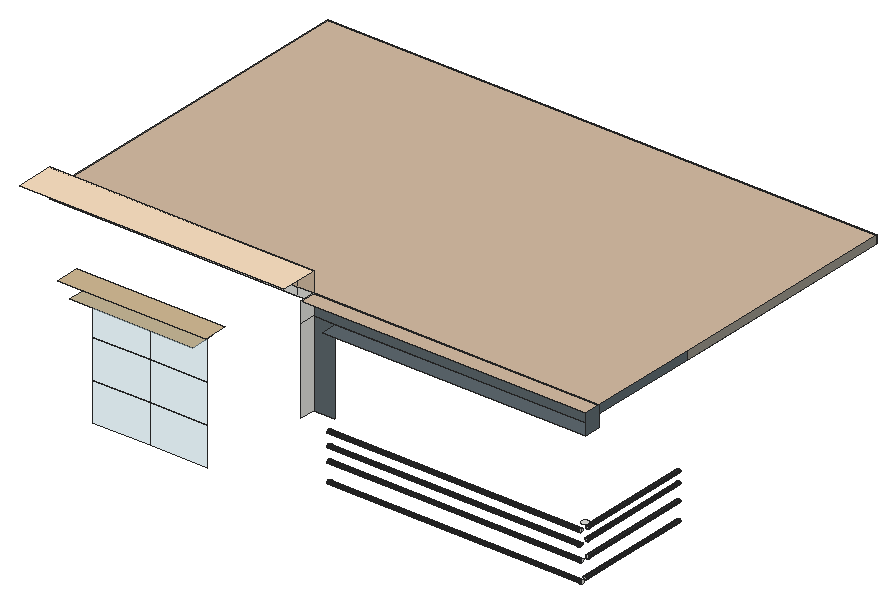
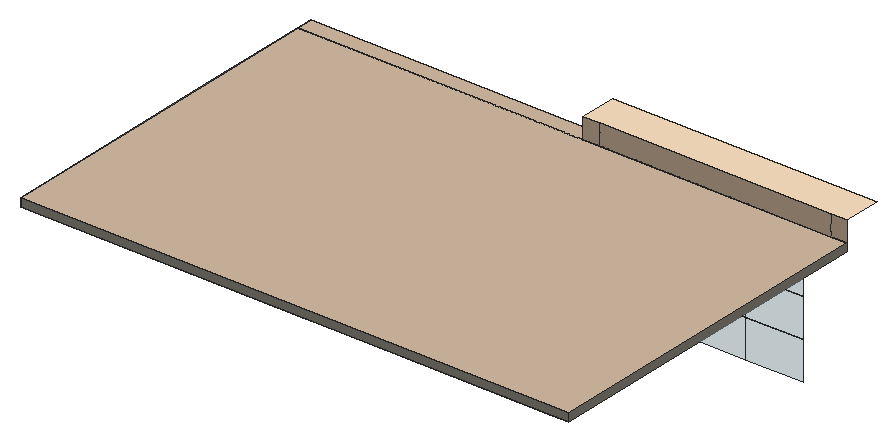
# SketchUp Ruby script. Lengths in inches.
U = 1.inch
M = Sketchup.active_model
def pt(a) = Geom::Point3d.new(a.map { |v| v * U })
def face(e, loops, mat)
  f = e.add_face(loops[0].map { |a| pt(a) })
  loops[1..].each { |l| e.add_face(l.map { |a| pt(a) }).erase! }
  f.material = f.back_material = mat if mat
  f
end
# faces: each face lists its corners as indices into pts; further lists are holes
def faces(e, pts, list, mat = nil) = list.each { |f| face(e, (f[0].is_a?(Array) ? f : [f]).map { |l| l.map { |i| pts[i] } }, mat) }
# xy, xz, yz: faces in a plane at the given z, y or x. An outline is a flat list of corners, or four numbers for a rectangle; further outlines are holes
def ring(l) = l.size == 4 ? [[l[0], l[1]], [l[2], l[1]], [l[2], l[3]], [l[0], l[3]]] : l.each_slice(2).to_a
def flat(e, list, mat, &to3) = list.each { |f| face(e, (f[0].is_a?(Array) ? f : [f]).map { |l| ring(l).map { |u, v| to3.(u, v) } }, mat) }
def xy(e, z, list, mat = nil) = flat(e, list, mat) { |x, y| [x, y, z] }
def xz(e, y, list, mat = nil) = flat(e, list, mat) { |x, z| [x, y, z] }
def yz(e, x, list, mat = nil) = flat(e, list, mat) { |y, z| [x, y, z] }
def lines(e, pts, list) = list.each { |a, b| e.add_line(pt(pts[a]), pt(pts[b])) }
# prism: a flat outline (further loops are holes) pulled along v
def prism(e, loops, v, mat = nil)
  f = face(e, loops, mat); d = Geom::Vector3d.new(v.map { |x| x * U })
  f.pushpull(f.normal.samedirection?(d) ? d.length : -d.length)
end
def box(e, o, s, mat = nil) = prism(e, [[o, [o[0] + s[0], o[1], o[2]], [o[0] + s[0], o[1] + s[1], o[2]], [o[0], o[1] + s[1], o[2]]]], [0, 0, s[2]], mat)
def at(x, y, z, deg = 0) = Geom::Transformation.translation(pt([x, y, z])) * Geom::Transformation.rotation(ORIGIN, Z_AXIS, deg.degrees)
def axes(o, x, y, z) = Geom::Transformation.new([*x, 0, *y, 0, *z, 0, *pt(o).to_a, 1])
def part(name) = M.definitions.add(name)
# library, detail: a bought-in or finely detailed component or shape, given as its bounding box
def library(name, o, s) = part(name).tap { |d| box(d.entities, o, s) }
def detail(e, o, s) = box(e.add_group.entities, o, s)
def put(e, d, t, mat = nil) = e.add_instance(d, t).tap { |i| i.material = mat if mat }
def group(e, t, mat = nil) = e.add_group.tap { |g| g.transformation = t; g.material = mat if mat }.entities
root = M.entities
M.materials.add("[0012_Bisque]").color = [255, 228, 196]
M.materials.add("[Color M07]").color = [58, 58, 58]
M.materials.add("[Formica Beige]").color = [211, 187, 149]
M.materials.add("[Formica Graystone]").color = [149, 146, 135]
M.materials.add("[Formica Laminate Light]").color = [213, 189, 164]
M.materials.add("[Formica Speckled Grey]").color = [94, 105, 111]
M.materials.add("[Quartz Light Brown]").color = [199, 184, 152]
M.materials.add("[Translucent Glass Safety]").color = [204, 235, 244]
M.materials["[Translucent Glass Safety]"].alpha = 0.5
c1 = library("Group\#1",[-0.5,-0.5,-0.1],[10.11,10.11,0.2])
c2 = library("Group\#2",[-0.5,-0.5,-0.1],[10.11,10.11,0.2])
c3 = library("Group\#3",[-0.5,-0.5,-0.1],[10.11,10.11,0.2])
c4 = library("Group\#4",[-0.5,-0.5,-0.1],[10.11,10.11,0.2])
xy(root,170.34,[[254.97,24.03,255.38,24.08,255.75,24.24,256.08,24.49,256.33,24.8125,256.48,25.19,256.54,25.59,256.48,26,256.33,26.375,256.08,26.7,255.75,26.95,255.38,27.1,254.97,27.16,254.57,27.1,254.19,26.95,253.87,26.7,253.62,26.375,253.46,26,253.41,25.59,253.46,25.19,253.62,24.8125,253.87,24.49,254.19,24.24,254.57,24.08]])
xy(root,197.75,[[32.29,0,90.53,11.1875]],"[Quartz Light Brown]")
xy(root,203.54,[[26.5,0,96.3125,11.1875]],"[Formica Beige]")
xy(root,210.1875,[[134.6,21.1875,259.04,28.73]],"[Formica Speckled Grey]")
xy(root,216.125,[[0,28.73,7.54,80.93],[7.54,28.73,116.61,80.93],[116.61,28.73,124.35,80.93],[0,80.93,7.54,89.9],[7.54,80.93,116.61,89.9],
  [116.61,80.93,124.35,89.9],[124.35,80.93,251.5,89.9],[251.5,80.93,259.04,89.9],[0,89.9,7.54,192.39],[7.54,89.9,116.61,184.85],
  [116.61,89.9,124.35,184.85],[124.35,89.9,251.5,184.85],[251.5,89.9,259.04,184.85],[7.54,184.85,116.61,192.39],[116.61,184.85,124.35,192.39],
  [124.35,184.85,259.04,192.39]])
xy(root,216.125,[[124.35,28.73,259.04,80.93]],"[Formica Speckled Grey]")
xy(root,219.875,[[124.35,21.1875,259.04,28.73],[0,28.73,259.04,192.39]],"[Formica Laminate Light]")
xy(root,229.5,[[0,11.1875,124.35,28.73]],"[0012_Bisque]")
xz(root,11.1875,[[34.45,140.9,61.41,159.07],[61.41,140.9,88.37,159.07],[34.45,159.07,61.41,177.24],[61.41,159.07,88.37,177.24],[34.45,177.24,61.41,195.59],
  [61.41,177.24,88.37,195.59]],"[Translucent Glass Safety]")
xz(root,25.59,[[254.99,145.96,255.2,145.99,255.39,146.07,255.5625,146.2,255.69,146.37,255.77,146.5625,255.8,146.77,255.77,146.98,255.69,147.18,255.5625,147.35,255.39,147.48,255.2,147.56,254.99,147.58,254.78,147.56,254.58,147.48,254.41,147.35,254.28,147.18,254.2,146.98,254.18,146.77,254.2,146.5625,254.28,146.37,254.41,146.2,254.58,146.07,254.78,145.99]])
xz(root,26.7,[[254.99,161.79,255.2,161.81,255.39,161.9,255.5625,162.03,255.69,162.19,255.77,162.39,255.8,162.6,255.77,162.81,255.69,163.01,255.5625,163.17,255.39,163.3,255.2,163.38,254.99,163.41,254.78,163.38,254.58,163.3,254.41,163.17,254.28,163.01,254.2,162.81,254.18,162.6,254.2,162.39,254.28,162.19,254.41,162.03,254.58,161.9,254.78,161.81]])
xz(root,26.99,[[254.99,166.97,255.2,167,255.39,167.08,255.5625,167.21,255.69,167.38,255.77,167.58,255.8,167.79,255.77,168,255.69,168.19,255.5625,168.36,255.39,168.49,255.2,168.57,254.99,168.6,254.78,168.57,254.58,168.49,254.41,168.36,254.28,168.19,254.2,168,254.18,167.79,254.2,167.58,254.28,167.38,254.41,167.21,254.58,167.08,254.78,167]])
xz(root,27.05,[[254.99,154.29,255.2,154.31,255.39,154.4,255.5625,154.53,255.69,154.69,255.77,154.89,255.8,155.1,255.77,155.31,255.69,155.51,255.5625,155.67,255.39,155.8,255.2,155.88,254.99,155.91,254.78,155.88,254.58,155.8,254.41,155.67,254.28,155.51,254.2,155.31,254.18,155.1,254.2,154.89,254.28,154.69,254.41,154.53,254.58,154.4,254.78,154.31]])
xz(root,28.73,[[0,216.125,116.61,219.875],[116.61,216.125,124.35,219.875],[124.35,216.125,259.04,219.875]])
xz(root,28.73,[[0,219.875,7.54,229.5],[7.54,219.875,116.61,229.5],[116.61,219.875,124.35,229.5]],"[Formica Laminate Light]")
xz(root,28.73,[[124.35,170.34,134.6,210.1875],[124.35,210.1875,259.04,216.125]],"[Formica Speckled Grey]")
xz(root,192.39,[[0,216.125,259.04,219.875]],"[Formica Graystone]")
yz(root,0,[[28.73,216.125,192.39,219.875]],"[Formica Graystone]")
yz(root,124.35,[[21.1875,170.34,28.73,210.1875],[21.1875,210.1875,28.73,219.875]])
yz(root,253.78,[[24.83,159.95,25.04,159.97,25.23,160.05,25.4,160.18,25.53,160.35,25.61,160.55,25.64,160.76,25.61,160.97,25.53,161.16,25.4,161.33,25.23,161.46,25.04,161.54,24.83,161.57,24.62,161.54,24.42,161.46,24.25,161.33,24.125,161.16,24.04,160.97,24.01,160.76,24.04,160.55,24.125,160.35,24.25,160.18,24.42,160.05,24.62,159.97]],"[Color M07]")
yz(root,253.87,[[24.83,166.07,25.04,166.1,25.23,166.18,25.4,166.31,25.53,166.48,25.61,166.67,25.64,166.88,25.61,167.09,25.53,167.29,25.4,167.46,25.23,167.59,25.04,167.67,24.83,167.7,24.62,167.67,24.49,167.62,24.49,166.15,24.62,166.1],[24.49,166.15,24.49,167.62,24.42,167.59,24.25,167.46,24.125,167.29,24.04,167.09,24.01,166.88,24.04,166.67,24.125,166.48,24.25,166.31,24.42,166.18]])
yz(root,254.19,[[24.83,153.38,25.04,153.41,25.23,153.49,25.4,153.62,25.53,153.79,25.61,153.99,25.64,154.2,25.61,154.41,25.53,154.6,25.4,154.77,25.23,154.9,25.04,154.98,24.83,155.01,24.62,154.98,24.42,154.9,24.25,154.77,24.24,154.75,24.24,153.64,24.25,153.62,24.42,153.49,24.62,153.41],[24.24,153.64,24.24,154.75,24.125,154.6,24.04,154.41,24.01,154.2,24.04,153.99,24.125,153.79]])
yz(root,254.57,[[24.83,144.63,25.04,144.66,25.23,144.74,25.4,144.87,25.53,145.04,25.61,145.24,25.64,145.45,25.61,145.66,25.53,145.85,25.4,146.02,25.23,146.15,25.04,146.23,24.83,146.26,24.62,146.23,24.42,146.15,24.25,146.02,24.125,145.85,24.08,145.76,24.08,145.13,24.125,145.04,24.25,144.87,24.42,144.74,24.62,144.66]])
yz(root,254.57,[[24.08,145.13,24.08,145.76,24.04,145.66,24.01,145.45,24.04,145.24]],"[Color M07]")
yz(root,259.04,[[80.93,216.125,192.39,219.875]],"[Formica Graystone]")
yz(root,259.04,[[21.1875,210.1875,28.73,219.875],[28.73,216.125,80.93,219.875]],"[Formica Speckled Grey]")
p = [[254.57,24.62,144.66],[134.6,24.62,144.66],[134.6,24.83,144.63],[254.57,24.83,144.63],[134.6,25.04,144.66],[254.57,25.04,144.66],
  [254.57,24.25,144.87],[134.6,24.25,144.87],[134.6,24.42,144.74],[254.57,24.42,144.74],[134.6,25.23,144.74],[254.57,25.23,144.74],
  [134.6,25.4,144.87],[254.57,25.4,144.87],[254.57,24.125,145.04],[134.6,24.125,145.04],[134.6,25.53,145.04],[254.57,25.53,145.04],
  [254.57,24.04,145.24],[134.6,24.04,145.24],[254.57,24.08,145.13],[134.6,25.61,145.24],[254.57,25.61,145.24],[254.57,24.01,145.45],
  [134.6,24.01,145.45],[134.6,25.64,145.45],[254.57,25.64,145.45],[254.57,24.04,145.66],[134.6,24.04,145.66],[134.6,25.61,145.66],
  [254.57,25.61,145.66],[254.57,24.125,145.85],[134.6,24.125,145.85],[254.57,24.08,145.76],[134.6,25.53,145.85],[254.57,25.53,145.85],
  [254.57,24.25,146.02],[134.6,24.25,146.02],[134.6,25.4,146.02],[254.57,25.4,146.02],[254.57,24.42,146.15],[134.6,24.42,146.15],
  [134.6,25.23,146.15],[254.57,25.23,146.15],[254.58,80.93,146.07],[254.78,80.93,145.99],[254.78,25.59,145.99],[254.58,25.59,146.07],
  [254.99,80.93,145.96],[254.99,25.59,145.96],[255.2,80.93,145.99],[255.2,25.59,145.99],[255.39,80.93,146.07],[255.39,25.59,146.07],
  [254.57,24.62,146.23],[134.6,24.62,146.23],[134.6,25.04,146.23],[254.57,25.04,146.23],[254.41,80.93,146.2],[254.41,25.59,146.2],
  [255.5625,80.93,146.2],[255.5625,25.59,146.2],[254.57,24.83,146.26],[134.6,24.83,146.26],[254.28,80.93,146.37],[254.28,25.59,146.37],
  [255.69,80.93,146.37],[255.69,25.59,146.37],[254.2,80.93,146.5625],[254.2,25.59,146.5625],[255.77,80.93,146.5625],[255.77,25.59,146.5625],
  [254.18,80.93,146.77],[254.18,25.59,146.77],[255.8,80.93,146.77],[255.8,25.59,146.77],[254.2,80.93,146.98],[254.2,25.59,146.98],
  [255.77,80.93,146.98],[255.77,25.59,146.98],[254.28,80.93,147.18],[254.28,25.59,147.18],[255.69,80.93,147.18],[255.69,25.59,147.18],
  [254.41,80.93,147.35],[254.41,25.59,147.35],[255.5625,80.93,147.35],[255.5625,25.59,147.35],[254.58,80.93,147.48],[254.58,25.59,147.48],
  [255.39,80.93,147.48],[255.39,25.59,147.48],[254.78,80.93,147.56],[254.78,25.59,147.56],[255.2,80.93,147.56],[255.2,25.59,147.56],
  [254.99,80.93,147.58],[254.99,25.59,147.58],[254.19,24.42,153.49],[134.6,24.42,153.49],[134.6,24.62,153.41],[254.19,24.62,153.41],
  [134.6,24.83,153.38],[254.19,24.83,153.38],[134.6,25.04,153.41],[254.19,25.04,153.41],[134.6,25.23,153.49],[254.19,25.23,153.49],
  [254.19,24.25,153.62],[134.6,24.25,153.62],[134.6,25.4,153.62],[254.19,25.4,153.62],[254.19,24.125,153.79],[134.6,24.125,153.79],
  [254.19,24.24,153.64],[134.6,25.53,153.79],[254.19,25.53,153.79],[254.19,24.04,153.99],[134.6,24.04,153.99],[134.6,25.61,153.99],
  [254.19,25.61,153.99],[254.19,24.01,154.2],[134.6,24.01,154.2],[134.6,25.64,154.2],[254.19,25.64,154.2],[254.19,24.04,154.41],
  [134.6,24.04,154.41],[134.6,25.61,154.41],[254.19,25.61,154.41],[254.58,80.93,154.4],[254.78,80.93,154.31],[254.78,27.05,154.31],
  [254.58,27.05,154.4],[254.99,80.93,154.29],[254.99,27.05,154.29],[255.2,80.93,154.31],[255.2,27.05,154.31],[255.39,80.93,154.4],
  [255.39,27.05,154.4],[254.19,24.125,154.6],[134.6,24.125,154.6],[134.6,25.53,154.6],[254.19,25.53,154.6],[254.41,80.93,154.53],
  [254.41,27.05,154.53],[255.5625,80.93,154.53],[255.5625,27.05,154.53],[254.28,80.93,154.69],[254.28,27.05,154.69],[255.69,80.93,154.69],
  [255.69,27.05,154.69],[254.19,24.25,154.77],[134.6,24.25,154.77],[254.19,24.24,154.75],[134.6,25.4,154.77],[254.19,25.4,154.77],
  [254.2,80.93,154.89],[254.2,27.05,154.89],[255.77,80.93,154.89],[255.77,27.05,154.89],[254.19,24.42,154.9],[134.6,24.42,154.9],
  [134.6,25.23,154.9],[254.19,25.23,154.9],[254.19,24.62,154.98],[134.6,24.62,154.98],[134.6,25.04,154.98],[254.19,25.04,154.98],
  [254.18,80.93,155.1],[254.18,27.05,155.1],[255.8,80.93,155.1],[255.8,27.05,155.1],[254.19,24.83,155.01],[134.6,24.83,155.01],
  [254.2,80.93,155.31],[254.2,27.05,155.31],[255.77,80.93,155.31],[255.77,27.05,155.31],[254.28,80.93,155.51],[254.28,27.05,155.51],
  [255.69,80.93,155.51],[255.69,27.05,155.51],[254.41,80.93,155.67],[254.41,27.05,155.67],[255.5625,80.93,155.67],[255.5625,27.05,155.67],
  [254.58,80.93,155.8],[254.58,27.05,155.8],[255.39,80.93,155.8],[255.39,27.05,155.8],[254.78,80.93,155.88],[254.78,27.05,155.88],
  [255.2,80.93,155.88],[255.2,27.05,155.88],[254.99,80.93,155.91],[254.99,27.05,155.91],[253.78,24.62,159.97],[134.6,24.62,159.97],
  [134.6,24.83,159.95],[253.78,24.83,159.95],[134.6,25.04,159.97],[253.78,25.04,159.97],[253.78,24.42,160.05],[134.6,24.42,160.05],
  [134.6,25.23,160.05],[253.78,25.23,160.05],[253.78,24.25,160.18],[134.6,24.25,160.18],[134.6,25.4,160.18],[253.78,25.4,160.18],
  [253.78,24.125,160.35],[134.6,24.125,160.35],[134.6,25.53,160.35],[253.78,25.53,160.35],[253.78,24.04,160.55],[134.6,24.04,160.55],
  [134.6,25.61,160.55],[253.78,25.61,160.55],[253.78,24.01,160.76],[134.6,24.01,160.76],[134.6,25.64,160.76],[253.78,25.64,160.76],
  [253.78,24.04,160.97],[134.6,24.04,160.97],[134.6,25.61,160.97],[253.78,25.61,160.97],[253.78,24.125,161.16],[134.6,24.125,161.16],
  [134.6,25.53,161.16],[253.78,25.53,161.16],[253.78,24.25,161.33],[134.6,24.25,161.33],[134.6,25.4,161.33],[253.78,25.4,161.33],
  [253.78,24.42,161.46],[134.6,24.42,161.46],[134.6,25.23,161.46],[253.78,25.23,161.46],[253.78,24.62,161.54],[134.6,24.62,161.54],
  [253.78,24.83,161.57],[134.6,24.83,161.57],[253.78,25.04,161.54],[134.6,25.04,161.54],[254.58,80.93,161.9],[254.78,80.93,161.81],
  [254.78,26.7,161.81],[254.58,26.7,161.9],[254.99,80.93,161.79],[254.99,26.7,161.79],[255.2,80.93,161.81],[255.2,26.7,161.81],
  [255.39,80.93,161.9],[255.39,26.7,161.9],[254.41,80.93,162.03],[254.41,26.7,162.03],[255.5625,80.93,162.03],[255.5625,26.7,162.03],
  [254.28,80.93,162.19],[254.28,26.7,162.19],[255.69,80.93,162.19],[255.69,26.7,162.19],[254.2,80.93,162.39],[254.2,26.7,162.39],
  [255.77,80.93,162.39],[255.77,26.7,162.39],[254.18,80.93,162.6],[254.18,26.7,162.6],[255.8,80.93,162.6],[255.8,26.7,162.6],
  [254.2,80.93,162.81],[254.2,26.7,162.81],[255.77,80.93,162.81],[255.77,26.7,162.81],[254.28,80.93,163.01],[254.28,26.7,163.01],
  [255.69,80.93,163.01],[255.69,26.7,163.01],[254.41,80.93,163.17],[254.41,26.7,163.17],[255.5625,80.93,163.17],[255.5625,26.7,163.17],
  [254.58,80.93,163.3],[254.58,26.7,163.3],[255.39,80.93,163.3],[255.39,26.7,163.3],[254.78,80.93,163.38],[254.78,26.7,163.38],
  [255.2,80.93,163.38],[255.2,26.7,163.38],[254.99,80.93,163.41],[254.99,26.7,163.41],[253.87,24.42,166.18],[134.6,24.42,166.18],
  [134.6,24.62,166.1],[253.87,24.62,166.1],[253.87,24.49,166.15],[134.6,24.83,166.07],[253.87,24.83,166.07],[134.6,25.04,166.1],
  [253.87,25.04,166.1],[134.6,25.23,166.18],[253.87,25.23,166.18],[253.87,24.25,166.31],[134.6,24.25,166.31],[134.6,25.4,166.31],
  [253.87,25.4,166.31],[253.87,24.125,166.48],[134.6,24.125,166.48],[134.6,25.53,166.48],[253.87,25.53,166.48],[253.87,24.04,166.67],
  [134.6,24.04,166.67],[134.6,25.61,166.67],[253.87,25.61,166.67],[253.87,24.01,166.88],[134.6,24.01,166.88],[134.6,25.64,166.88],
  [253.87,25.64,166.88],[253.87,24.04,167.09],[134.6,24.04,167.09],[134.6,25.61,167.09],[253.87,25.61,167.09],[254.58,80.93,167.08],
  [254.78,80.93,167],[254.78,26.99,167],[254.58,26.99,167.08],[254.99,80.93,166.97],[254.99,26.99,166.97],[255.2,80.93,167],
  [255.2,26.99,167],[255.39,80.93,167.08],[255.39,26.99,167.08],[253.87,24.125,167.29],[134.6,24.125,167.29],[134.6,25.53,167.29],
  [253.87,25.53,167.29],[254.41,80.93,167.21],[254.41,26.99,167.21],[255.5625,80.93,167.21],[255.5625,26.99,167.21],[254.28,80.93,167.38],
  [254.28,26.99,167.38],[255.69,80.93,167.38],[255.69,26.99,167.38],[253.87,24.25,167.46],[134.6,24.25,167.46],[134.6,25.4,167.46],
  [253.87,25.4,167.46],[254.2,80.93,167.58],[254.2,26.99,167.58],[255.77,80.93,167.58],[255.77,26.99,167.58],[253.87,24.42,167.59],
  [134.6,24.42,167.59],[134.6,25.23,167.59],[253.87,25.23,167.59],[253.87,24.62,167.67],[134.6,24.62,167.67],[253.87,24.49,167.62],
  [134.6,25.04,167.67],[253.87,25.04,167.67],[254.18,80.93,167.79],[254.18,26.99,167.79],[255.8,80.93,167.79],[255.8,26.99,167.79],
  [253.87,24.83,167.7],[134.6,24.83,167.7],[254.2,80.93,168],[254.2,26.99,168],[255.77,80.93,168],[255.77,26.99,168],
  [254.28,80.93,168.19],[254.28,26.99,168.19],[255.69,80.93,168.19],[255.69,26.99,168.19],[254.41,80.93,168.36],[254.41,26.99,168.36],
  [255.5625,80.93,168.36],[255.5625,26.99,168.36],[254.58,80.93,168.49],[254.58,26.99,168.49],[255.39,80.93,168.49],[255.39,26.99,168.49],
  [254.78,80.93,168.57],[254.78,26.99,168.57],[255.2,80.93,168.57],[255.2,26.99,168.57],[254.99,80.93,168.6],[254.99,26.99,168.6]]
faces(root,p,[[0,1,2,3],[3,2,4,5],[6,7,8,9],[9,8,1,0],[5,4,10,11],[11,10,12,13],[14,15,7,6],[13,12,16,17],
  [18,19,15,14,20],[17,16,21,22],[23,24,19,18],[22,21,25,26],[27,28,24,23],[26,25,29,30],[31,32,28,27,33],[30,29,34,35],
  [36,37,32,31],[35,34,38,39],[40,41,37,36],[39,38,42,43],[44,45,46,47],[45,48,49,46],[48,50,51,49],[50,52,53,51],
  [54,55,41,40],[43,42,56,57],[58,44,47,59],[52,60,61,53],[62,63,55,54],[57,56,63,62],[64,58,59,65],[60,66,67,61],
  [68,64,65,69],[66,70,71,67],[72,68,69,73],[70,74,75,71],[76,72,73,77],[74,78,79,75],[80,76,77,81],[78,82,83,79],
  [84,80,81,85],[82,86,87,83],[88,84,85,89],[86,90,91,87],[92,88,89,93],[90,94,95,91],[96,92,93,97],[94,96,97,95],
  [98,99,100,101],[101,100,102,103],[103,102,104,105],[105,104,106,107],[108,109,99,98],[107,106,110,111],[112,113,109,108,114],[111,110,115,116],
  [117,118,113,112],[116,115,119,120],[121,122,118,117],[120,119,123,124],[125,126,122,121],[124,123,127,128],[129,130,131,132],[130,133,134,131],
  [133,135,136,134],[135,137,138,136],[139,140,126,125],[128,127,141,142],[143,129,132,144],[137,145,146,138],[147,143,144,148],[145,149,150,146],
  [151,152,140,139,153],[142,141,154,155],[156,147,148,157],[149,158,159,150],[160,161,152,151],[155,154,162,163],[164,165,161,160],[163,162,166,167],
  [168,156,157,169],[158,170,171,159],[172,173,165,164],[167,166,173,172],[174,168,169,175],[170,176,177,171],[178,174,175,179],[176,180,181,177],
  [182,178,179,183],[180,184,185,181],[186,182,183,187],[184,188,189,185],[190,186,187,191],[188,192,193,189],[194,190,191,195],[192,194,195,193],
  [196,197,198,199],[199,198,200,201],[202,203,197,196],[201,200,204,205],[206,207,203,202],[205,204,208,209],[210,211,207,206],[209,208,212,213],
  [214,215,211,210],[213,212,216,217],[218,219,215,214],[217,216,220,221],[222,223,219,218],[221,220,224,225],[226,227,223,222],[225,224,228,229],
  [230,231,227,226],[229,228,232,233],[234,235,231,230],[233,232,236,237],[238,239,235,234],[240,241,239,238],[242,243,241,240],[237,236,243,242],
  [244,245,246,247],[245,248,249,246],[248,250,251,249],[250,252,253,251],[254,244,247,255],[252,256,257,253],[258,254,255,259],[256,260,261,257],
  [262,258,259,263],[260,264,265,261],[266,262,263,267],[264,268,269,265],[270,266,267,271],[268,272,273,269],[274,270,271,275],[272,276,277,273],
  [278,274,275,279],[276,280,281,277],[282,278,279,283],[280,284,285,281],[286,282,283,287],[284,288,289,285],[290,286,287,291],[288,290,291,289],
  [292,293,294,295,296],[295,294,297,298],[298,297,299,300],[300,299,301,302],[303,304,293,292],[302,301,305,306],[307,308,304,303],[306,305,309,310],
  [311,312,308,307],[310,309,313,314],[315,316,312,311],[314,313,317,318],[319,320,316,315],[318,317,321,322],[323,324,325,326],[324,327,328,325],
  [327,329,330,328],[329,331,332,330],[333,334,320,319],[322,321,335,336],[337,323,326,338],[331,339,340,332],[341,337,338,342],[339,343,344,340],
  [345,346,334,333],[336,335,347,348],[349,341,342,350],[343,351,352,344],[353,354,346,345],[348,347,355,356],[357,358,354,353,359],[356,355,360,361],
  [362,349,350,363],[351,364,365,352],[366,367,358,357],[361,360,367,366],[368,362,363,369],[364,370,371,365],[372,368,369,373],[370,374,375,371],
  [376,372,373,377],[374,378,379,375],[380,376,377,381],[378,382,383,379],[384,380,381,385],[382,386,387,383],[388,384,385,389],[386,388,389,387]],"[Color M07]")
put(root,c1,axes([159.73,45.75,216.125],[-1,0,0],[0,1,0],[0,0,-1]))
put(root,c2,axes([155.85,65,216.125],[-1,0,0],[0,1,0],[0,0,-1]))
put(root,c3,axes([214.29,45.75,216.125],[-1,0,0],[0,1,0],[0,0,-1]))
put(root,c4,axes([214.29,65,216.125],[-1,0,0],[0,1,0],[0,0,-1]))
